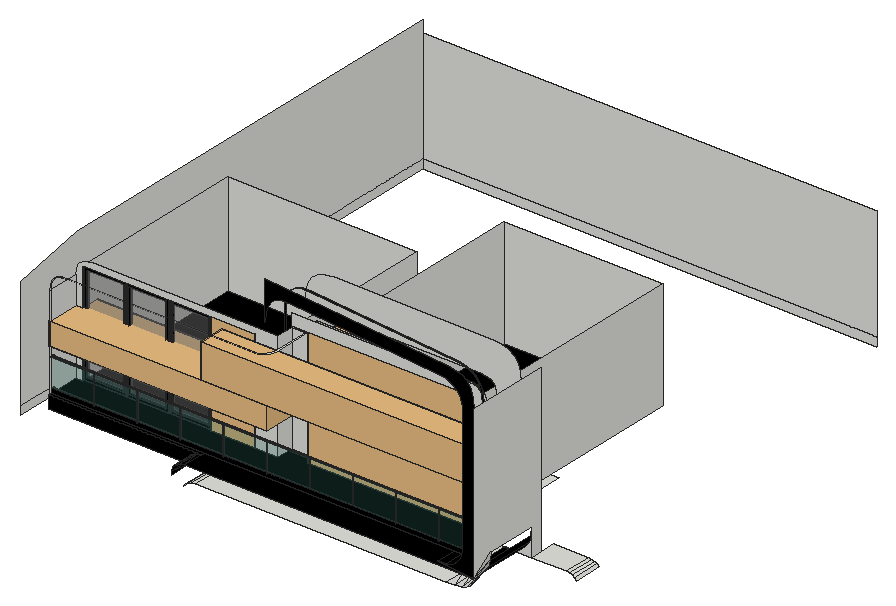
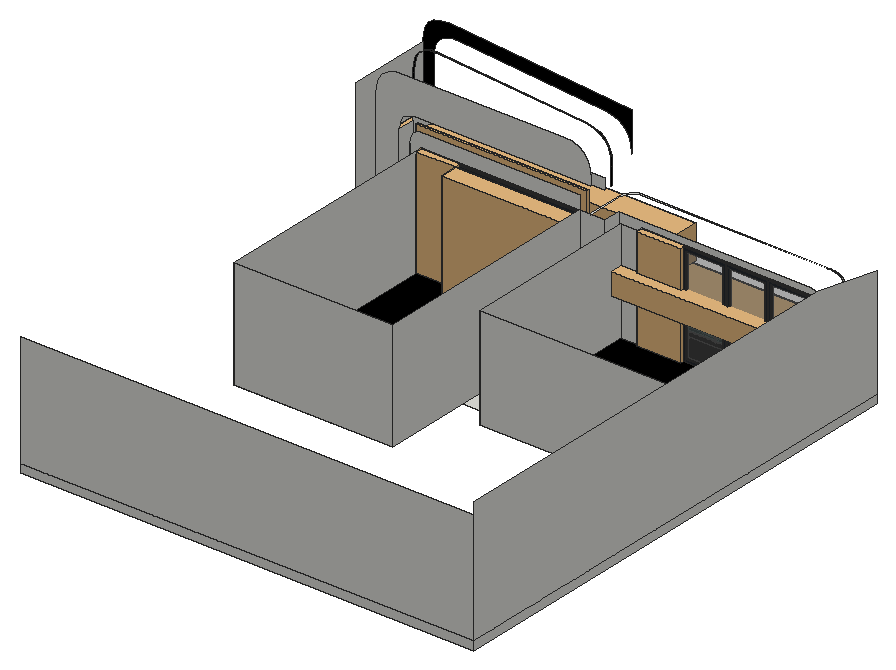
# SketchUp Ruby script. Lengths in inches.
U = 1.inch
M = Sketchup.active_model
def pt(a) = Geom::Point3d.new(a.map { |v| v * U })
def face(e, loops, mat)
  f = e.add_face(loops[0].map { |a| pt(a) })
  loops[1..].each { |l| e.add_face(l.map { |a| pt(a) }).erase! }
  f.material = f.back_material = mat if mat
  f
end
# faces: each face lists its corners as indices into pts; further lists are holes
def faces(e, pts, list, mat = nil) = list.each { |f| face(e, (f[0].is_a?(Array) ? f : [f]).map { |l| l.map { |i| pts[i] } }, mat) }
# xy, xz, yz: faces in a plane at the given z, y or x. An outline is a flat list of corners, or four numbers for a rectangle; further outlines are holes
def ring(l) = l.size == 4 ? [[l[0], l[1]], [l[2], l[1]], [l[2], l[3]], [l[0], l[3]]] : l.each_slice(2).to_a
def flat(e, list, mat, &to3) = list.each { |f| face(e, (f[0].is_a?(Array) ? f : [f]).map { |l| ring(l).map { |u, v| to3.(u, v) } }, mat) }
def xy(e, z, list, mat = nil) = flat(e, list, mat) { |x, y| [x, y, z] }
def xz(e, y, list, mat = nil) = flat(e, list, mat) { |x, z| [x, y, z] }
def yz(e, x, list, mat = nil) = flat(e, list, mat) { |y, z| [x, y, z] }
def lines(e, pts, list) = list.each { |a, b| e.add_line(pt(pts[a]), pt(pts[b])) }
# prism: a flat outline (further loops are holes) pulled along v
def prism(e, loops, v, mat = nil)
  f = face(e, loops, mat); d = Geom::Vector3d.new(v.map { |x| x * U })
  f.pushpull(f.normal.samedirection?(d) ? d.length : -d.length)
end
def box(e, o, s, mat = nil) = prism(e, [[o, [o[0] + s[0], o[1], o[2]], [o[0] + s[0], o[1] + s[1], o[2]], [o[0], o[1] + s[1], o[2]]]], [0, 0, s[2]], mat)
def at(x, y, z, deg = 0) = Geom::Transformation.translation(pt([x, y, z])) * Geom::Transformation.rotation(ORIGIN, Z_AXIS, deg.degrees)
def axes(o, x, y, z) = Geom::Transformation.new([*x, 0, *y, 0, *z, 0, *pt(o).to_a, 1])
def part(name) = M.definitions.add(name)
# library, detail: a bought-in or finely detailed component or shape, given as its bounding box
def library(name, o, s) = part(name).tap { |d| box(d.entities, o, s) }
def detail(e, o, s) = box(e.add_group.entities, o, s)
def put(e, d, t, mat = nil) = e.add_instance(d, t).tap { |i| i.material = mat if mat }
def group(e, t, mat = nil) = e.add_group.tap { |g| g.transformation = t; g.material = mat if mat }.entities
root = M.entities
M.materials.add("Glass Railing Color").color = [198, 198, 198]
M.materials.add("Railing Glass").color = [63, 150, 137]
M.materials["Railing Glass"].alpha = 0.13
M.materials.add("[0130_Gainsboro]").color = [39, 45, 50]
M.materials.add("[Color M00]").color = [255, 255, 255]
M.materials.add("[Color M09]").color = [0, 0, 0]
M.materials.add("[Color M09]1").color = [0, 0, 0]
M.materials.add("[Translucent Glass Gray]1").color = [128, 128, 128]
M.materials["[Translucent Glass Gray]1"].alpha = 0.5
M.materials.add("[Wood Veneer 02]").color = [190, 128, 91]
c1 = library("door by lz",[5.91,-4.92,0],[35.43,6.61,78.74])
c2 = part("Glazed door panel")
xy(c2.entities,0,[[0,-0.98,43.07,0],[0,0,43.07,1.4]],"[0130_Gainsboro]")
xy(c2.entities,0.3,[[0.3,-1.43,42.77,-0.98]],"[0130_Gainsboro]")
xy(c2.entities,2.95,[[2.95,-0.63,40.12,0],[2.95,0,40.12,0.64],[2.95,0.64,40.12,1.4]],"[0130_Gainsboro]")
xy(c2.entities,2.95,[[2.95,-1.43,40.12,-0.63]],"[Color M09]")
xy(c2.entities,3.54,[[3.54,0,39.53,0.64]],"[0130_Gainsboro]")
xy(c2.entities,3.54,[[3.54,-0.63,39.53,0]],"[Color M09]")
xy(c2.entities,111.8125,[[3.54,0,39.53,0.64]],"[0130_Gainsboro]")
xy(c2.entities,111.8125,[[3.54,-0.63,39.53,0]],"[Color M09]")
xy(c2.entities,112.4,[[2.95,-0.63,40.12,0],[2.95,0,40.12,0.64],[2.95,0.64,40.12,1.4]],"[0130_Gainsboro]")
xy(c2.entities,112.4,[[2.95,-1.43,40.12,-0.63]],"[Color M09]")
xy(c2.entities,115.05,[[0.3,-1.43,42.77,-0.98]],"[0130_Gainsboro]")
xy(c2.entities,115.35,[[0,-0.98,43.07,0],[0,0,43.07,1.4]],"[0130_Gainsboro]")
xz(c2.entities,-1.43,[[[0.3,0.3,42.77,115.05],[2.95,2.95,40.12,112.4]]],"[Color M09]")
xz(c2.entities,-0.98,[[[0,0,43.07,115.35],[0.3,0.3,42.77,115.05]]],"[Color M00]")
xz(c2.entities,-0.63,[[[2.95,2.95,40.12,112.4],[3.54,3.54,39.53,111.8125]]],"[Color M09]")
xz(c2.entities,0,[[[0,0,43.07,115.35],[2.95,2.95,40.12,112.4]],[[2.95,2.95,40.12,112.4],[3.54,3.54,39.53,111.8125]]],"[0130_Gainsboro]")
xz(c2.entities,0,[[3.54,3.54,39.53,111.8125]],"[Translucent Glass Gray]1")
xz(c2.entities,0.64,[[[2.95,2.95,40.12,112.4],[3.54,3.54,39.53,111.8125]]],"[0130_Gainsboro]")
xz(c2.entities,1.4,[[[0,0,43.07,115.35],[2.95,2.95,40.12,112.4]]],"[0130_Gainsboro]")
yz(c2.entities,0,[[-0.98,0,0,115.35],[0,0,1.4,115.35]],"[0130_Gainsboro]")
yz(c2.entities,0.3,[[-1.43,0.3,-0.98,115.05]],"[Color M00]")
yz(c2.entities,2.95,[[-0.63,2.95,0,112.4],[0,2.95,0.64,112.4],[0.64,2.95,1.4,112.4]],"[0130_Gainsboro]")
yz(c2.entities,2.95,[[-1.43,2.95,-0.63,112.4]],"[Color M09]")
yz(c2.entities,3.54,[[0,3.54,0.64,111.8125]],"[0130_Gainsboro]")
yz(c2.entities,3.54,[[-0.63,3.54,0,111.8125]],"[Color M09]")
yz(c2.entities,39.53,[[0,3.54,0.64,111.8125]],"[0130_Gainsboro]")
yz(c2.entities,39.53,[[-0.63,3.54,0,111.8125]],"[Color M09]")
yz(c2.entities,40.12,[[-0.63,2.95,0,112.4],[0,2.95,0.64,112.4],[0.64,2.95,1.4,112.4]],"[0130_Gainsboro]")
yz(c2.entities,40.12,[[-1.43,2.95,-0.63,112.4]],"[Color M09]")
yz(c2.entities,42.77,[[-1.43,0.3,-0.98,115.05]],"[Color M00]")
yz(c2.entities,43.07,[[-0.98,0,0,115.35],[0,0,1.4,115.35]],"[0130_Gainsboro]")
c3 = part("Sliding glass doors")
put(c3.entities,c2,axes([90.57,1.43,0],[1.05148,0,0],[0,1,0],[0,0,1]),"[Color M09]")
put(c3.entities,c2,axes([0,1.43,0],[1.05148,0,0],[0,1,0],[0,0,1]))
put(c3.entities,c2,axes([45.29,1.43,0],[1.05148,0,0],[0,1,0],[0,0,1]))
c4 = library("Curtains",[0,0,0],[121.73,8.19,117.22])
c5 = part("Glass Rail Spacer")
box(c5.entities,[-0.5,-0.25,0],[1,0.5,1],"Glass Railing Color")
c6 = part("Group242\#1")
xz(c6.entities,0,[[-0.01,0,0.18,0.02,0.37,0.09,0.52,0.21,0.64,0.37,0.72,0.54,0.75,0.74,0.73,0.93,0.66,1.12,0.54,1.27,0.38,1.39,0.21,1.47,0.01,1.5,-0.18,1.48,-0.37,1.41,-0.52,1.29,-0.64,1.13,-0.72,0.96,-0.75,0.76,-0.73,0.57,-0.66,0.38,-0.54,0.23,-0.38,0.11,-0.21,0.03]],"Glass Railing Color")
xz(c6.entities,457,[[-0.01,0,-0.21,0.03,-0.38,0.11,-0.54,0.23,-0.66,0.38,-0.73,0.57,-0.75,0.76,-0.72,0.96,-0.64,1.13,-0.52,1.29,-0.37,1.41,-0.18,1.48,0.01,1.5,0.21,1.47,0.38,1.39,0.54,1.27,0.66,1.12,0.73,0.93,0.75,0.74,0.72,0.54,0.64,0.37,0.52,0.21,0.37,0.09,0.18,0.02]],"Glass Railing Color")
p = [[-0.38,0,0.11],[-0.38,457,0.11],[-0.21,457,0.03],[-0.21,0,0.03],[-0.01,457,0],[-0.01,0,0],
  [0.18,457,0.02],[0.18,0,0.02],[0.37,457,0.09],[0.37,0,0.09],[-0.54,0,0.23],[-0.54,457,0.23],
  [0.52,457,0.21],[0.52,0,0.21],[-0.66,0,0.38],[-0.66,457,0.38],[0.64,457,0.37],[0.64,0,0.37],
  [-0.73,0,0.57],[-0.73,457,0.57],[0.72,457,0.54],[0.72,0,0.54],[0.75,457,0.74],[0.75,0,0.74],
  [-0.75,0,0.76],[-0.75,457,0.76],[0.73,457,0.93],[0.73,0,0.93],[-0.72,0,0.96],[-0.72,457,0.96],
  [0.66,457,1.12],[0.66,0,1.12],[-0.64,0,1.13],[-0.64,457,1.13],[-0.52,0,1.29],[-0.52,457,1.29],
  [0.54,457,1.27],[0.54,0,1.27],[-0.37,0,1.41],[-0.37,457,1.41],[0.38,457,1.39],[0.38,0,1.39],
  [-0.18,0,1.48],[-0.18,457,1.48],[0.21,457,1.47],[0.21,0,1.47],[0.01,0,1.5],[0.01,457,1.5]]
faces(c6.entities,p,[[0,1,2,3],[3,2,4,5],[5,4,6,7],[7,6,8,9],[10,11,1,0],[9,8,12,13],[14,15,11,10],[13,12,16,17],
  [18,19,15,14],[17,16,20,21],[21,20,22,23],[24,25,19,18],[23,22,26,27],[28,29,25,24],[27,26,30,31],[32,33,29,28],
  [34,35,33,32],[31,30,36,37],[38,39,35,34],[37,36,40,41],[42,43,39,38],[41,40,44,45],[46,47,43,42],[45,44,47,46]],"[Color M09]1")
c7 = part("Group245\#1")
prism(c7.entities,[[[0.25,0,5],[0.25,0,4],[-0.25,0,4],[-0.25,0,5],[-0.5,0,5],[-0.5,0,0],[0.5,0,0],[0.5,0,5]]],[0,457,0],"[Color M09]1")
c8 = part("Group246\#1")
box(c8.entities,[-0.1875,0,0],[0.375,44.6,30],"Railing Glass")
c9 = part("Group247\#1")
box(c9.entities,[-0.1875,0,0],[0.375,44.6,30],"Railing Glass")
c10 = part("Group248\#1")
box(c10.entities,[-0.1875,0,0],[0.375,44.6,30],"Railing Glass")
c11 = part("Group249\#1")
box(c11.entities,[-0.1875,0,0],[0.375,44.6,30],"Railing Glass")
c12 = part("Group250\#1")
box(c12.entities,[-0.1875,0,0],[0.375,44.6,30],"Railing Glass")
c13 = part("Group251\#1")
box(c13.entities,[-0.1875,0,0],[0.375,44.6,30],"Railing Glass")
c14 = part("Group252\#1")
box(c14.entities,[-0.1875,0,0],[0.375,44.6,30],"Railing Glass")
c15 = part("Group253\#1")
box(c15.entities,[-0.1875,0,0],[0.375,44.6,30],"Railing Glass")
c16 = part("Group254\#1")
box(c16.entities,[-0.1875,0,0],[0.375,44.6,30],"Railing Glass")
c17 = part("Group255\#1")
box(c17.entities,[-0.1875,0,0],[0.375,44.6,30],"Railing Glass")
c18 = part("Glass Railing")
put(c18.entities,c5,at(0,0,4))
put(c18.entities,c5,at(45.6,0,4))
put(c18.entities,c5,at(91.2,0,4))
put(c18.entities,c5,at(136.8,0,4))
put(c18.entities,c5,at(182.4,0,4))
put(c18.entities,c5,at(228,0,4))
put(c18.entities,c5,at(273.6,0,4))
put(c18.entities,c5,at(319.2,0,4))
put(c18.entities,c5,at(364.8,0,4))
put(c18.entities,c5,at(410.4,0,4))
put(c18.entities,c5,at(456,0,4))
put(c18.entities,c6,at(-0.5,0,34,-90),"Glass Railing Color")
put(c18.entities,c7,at(-0.5,0,0,-90),"Glass Railing Color")
put(c18.entities,c8,at(0.5,0,4,-90),"Railing Glass")
put(c18.entities,c9,at(46.1,0,4,-90),"Railing Glass")
put(c18.entities,c10,at(91.7,0,4,-90),"Railing Glass")
put(c18.entities,c11,at(137.3,0,4,-90),"Railing Glass")
put(c18.entities,c12,at(182.9,0,4,-90),"Railing Glass")
put(c18.entities,c13,at(228.5,0,4,-90),"Railing Glass")
put(c18.entities,c14,at(274.1,0,4,-90),"Railing Glass")
put(c18.entities,c15,at(319.7,0,4,-90),"Railing Glass")
put(c18.entities,c16,at(365.3,0,4,-90),"Railing Glass")
put(c18.entities,c17,at(410.9,0,4,-90),"Railing Glass")
c19 = library("Mesh Light",[-0.5,-0.5,-0.1],[1,1,0.2])
c20 = library("Group\#5",[-0.5,-0.5,0],[180.91,2,130.125])
c21 = library("Mesh Light\#1",[-0.5,-0.5,-0.1],[1,1,0.2])
xy(root,143.7,[[967.75,260.875,1015.75,406.0625],[1027.75,260.875,1183.9375,406.0625]])
xy(root,144,[[795.4375,260.875,931.4375,467.3125]])
xy(root,150,[[963.61,202.125,1228.2,233.0625],[1228,233.0625,1228.2,234.0625],[963.61,234.0625,963.61,260.875,1196.71,260.875,1196.71,278.875,1228.2,278.875,1228.2,234.0625],[1257.4375,278.875,1294.21,307.9375]])
xy(root,150,[[789.4375,224.875,937.4375,260.875]],"[Color M09]")
xy(root,163.875,[[951.61,202.125,1257.4375,202.125,1216.2,206.05,1216.2,231.99,952.57,231.99,952.57,224.875,951.61,224.875],[789.4375,224.875,951.61,224.875,951.61,232.99,1216.2,232.99,1216.2,260.875,1209.4375,260.875,1209.4375,278.875,1197.4375,278.875,1197.4375,527.4375,1029.53,527.4375,1029.53,278.875,1003.53,278.875,1003.53,260.875,978.47,260.875,978.47,266.1,996.66,266.1,996.66,453.4375,796.3125,453.4375,796.3125,260.875,789.4375,260.875]],"[Color M09]")
xz(root,224.875,[[789.4375,150,937.4375,150,937.83,154.24,939.01,157.71,940.98,160.41,943.74,162.33,947.28,163.49,951.61,163.875,789.4375,163.875]],"[Color M09]")
xz(root,260.875,[[789.4375,163.875,796.3125,163.875,796.3125,272.125,978.47,272.125,978.47,163.875,1003.53,163.875,1003.53,279,806.73,279,801.45,278.52,797.125,277.08,793.76,274.68,791.36,271.3125,789.92,266.99,789.4375,261.71],[1209.4375,163.875,1216.2,163.875,1221.4375,164.35,1221.4375,288.5625,1220.95,293.89,1219.5,298.25,1217.08,301.64,1213.6875,304.0625,1209.33,305.52,1204,306,1018.27,306,1018.27,294,1194.29,294,1198.92,293.58,1202.71,292.32,1205.65,290.21,1207.75,287.27,1209.02,283.48,1209.4375,278.86]])
xz(root,266.1,[[978.47,163.875,996.66,272.125]])
xz(root,278.875,[[1228.2,150,1257.4375,150,1257.4375,179.24,1256.625,170.31,1254.1875,163,1250.13,157.31,1244.44,153.25,1237.13,150.8125],[1003.53,163.875,1029.53,279],[1197.4375,163.875,1209.4375,163.875,1209.4375,278.86,1209.02,283.48,1207.75,287.27,1205.65,290.21,1202.71,292.32,1198.92,293.58,1194.29,294,1029.53,294,1029.53,279,1197.4375,279],[1216.2,163.875,1221.4375,163.875,1221.4375,164.35],[1221.4375,164.35,1225.13,164.6875,1232.44,167.125,1238.13,171.19,1242.1875,176.87,1244.625,184.18,1245.4375,193.12,1245.4375,312.76,1244.625,321.69,1242.1875,329,1238.13,334.69,1232.44,338.75,1225.13,341.1875,1216.2,342,1047.51,342,1038.58,341.1875,1031.27,338.75,1025.58,334.69,1021.52,329,1019.09,321.69,1018.27,312.76,1018.27,306,1204,306,1209.33,305.52,1213.6875,304.0625,1217.08,301.64,1219.5,298.25,1220.95,293.89,1221.4375,288.5625]])
xz(root,453.4375,[[796.3125,163.875,996.66,272.125]])
xz(root,527.4375,[[1029.53,163.875,1197.4375,279]])
xz(root,734.875,[[777.4375,150,1257.4375,159],[777.4375,159,1257.4375,279]])
yz(root,777.4375,[[202.125,150,734.875,159],[202.125,159,202.125,276.71,278.875,291,734.875,291,734.875,159]])
yz(root,789.4375,[[227.5,163.875,260.875,261.71]])
yz(root,796.3125,[[260.875,163.875,453.4375,272.125]])
yz(root,978.47,[[260.875,163.875,266.1,272.125]])
yz(root,996.66,[[266.1,163.875,453.4375,272.125]])
yz(root,1003.53,[[260.875,163.875,278.875,279]])
yz(root,1029.53,[[278.875,163.875,527.4375,279]])
yz(root,1197.4375,[[278.875,163.875,527.4375,279]])
yz(root,1209.4375,[[260.875,163.875,268.8125,278.86],[269.8125,163.875,278.875,278.86]])
yz(root,1221.4375,[[260.875,164.35,278.875,288.5625]])
yz(root,1257.4375,[[278.875,150,290.7,150,290.7,324.76,202.125,324.76,202.125,163.875,224.875,179.24,278.875,179.24]])
p = [[951.01,202.125,143.7],[951.01,233.0625,143.7],[952.98,233.0625,146.46],[952.98,202.125,146.46],[952.98,260.875,146.46],[952.98,234.0625,146.46],
  [951.01,234.0625,143.7],[951.01,260.875,143.7],[1304.88,278.875,144.67],[1304.88,307.9375,144.67],[1303.21,307.9375,147],[1303.21,278.875,147],
  [955.74,233.0625,148.43],[955.74,202.125,148.43],[955.74,260.875,148.43],[955.74,234.0625,148.43],[1300.88,307.9375,148.67],[1300.88,278.875,148.67],
  [959.28,233.0625,149.61],[959.28,202.125,149.61],[959.28,260.875,149.61],[959.28,234.0625,149.61],[1297.88,307.9375,149.67],[1297.88,278.875,149.67],
  [963.61,233.0625,150],[963.61,202.125,150],[963.61,260.875,150],[963.61,234.0625,150],[937.4375,224.875,150],[937.4375,202.125,149.7],
  [937.83,202.125,154.03],[1294.21,307.9375,150],[1294.21,278.875,150],[937.83,224.875,154.24],[1228.2,202.125,150],[1228.2,224.875,150],
  [1237.13,202.125,150.39],[1237.13,224.875,150.8125],[1228.2,233.0625,150],[1228.2,234.0625,150],[1228.2,278.875,150],[1237.13,278.875,150.8125],
  [1244.44,202.125,151.54],[1244.44,224.875,153.25],[1244.44,278.875,153.25],[1250.13,202.125,153.47],[1250.13,224.875,157.31],[1250.13,278.875,157.31],
  [1254.1875,202.125,156.17],[939.01,202.125,157.58],[939.01,224.875,157.71],[1254.1875,224.875,163],[1256.625,202.125,159.64],[1254.1875,278.875,163],
  [940.98,202.125,160.33],[940.98,224.875,160.41],[1256.625,224.875,170.31],[1257.4375,202.125,163.875],[943.74,202.125,162.3],[943.74,224.875,162.33],
  [947.28,202.125,163.48],[947.28,224.875,163.49],[1256.625,278.875,170.31],[951.61,202.125,163.875],[951.61,224.875,163.875],[1257.4375,202.125,324.76],
  [1256.625,202.2,333.69],[1254.1875,202.43,341],[1250.13,202.82,346.69],[1244.44,203.36,350.75],[1237.13,204.06,353.1875],[1228.2,204.91,354],
  [1018.27,224.875,354],[1018.27,224.875,312.76],[1019.09,224.8,321.69],[1021.52,224.57,329],[1025.58,224.18,334.69],[1031.27,223.64,338.75],
  [1038.58,222.94,341.1875],[1047.51,222.09,342],[1216.2,206.05,342],[1225.13,205.2,341.1875],[1232.44,204.5,338.75],[1238.13,203.96,334.69],
  [1242.1875,203.58,329],[1244.625,203.34,321.69],[1245.4375,203.27,312.76],[1245.4375,203.27,193.12],[1244.625,203.34,184.18],[1242.1875,203.58,176.87],
  [1238.13,203.96,171.19],[1232.44,204.5,167.125],[1225.13,205.2,164.6875],[1216.2,206.05,163.875],[1257.4375,224.875,179.24],[1225.13,231.14,164.6875],
  [1216.2,231.99,163.875],[1216.2,260.875,163.875],[1216.2,232.99,163.875],[1225.13,232.14,164.6875],[1225.13,278.875,164.6875],[1221.4375,278.875,164.35],
  [1221.4375,260.875,164.35],[1216.2,278.875,163.875],[1232.44,230.44,167.125],[1232.44,231.44,167.125],[1232.44,278.875,167.125],[789.4375,226.5,150],
  [789.4375,226.5,163.875],[789.4375,227.5,150],[789.4375,227.5,163.875]]
faces(root,p,[[0,1,2,3],[4,5,6,7],[8,9,10,11],[3,2,12,13],[14,15,5,4],[11,10,16,17],[13,12,18,19],[20,21,15,14],
  [17,16,22,23],[19,18,24,25],[26,27,21,20],[23,22,31,32],[34,35,36],[35,37,36],[36,37,42],[37,43,42],
  [42,43,45],[43,46,45],[45,46,48],[46,51,48],[48,51,52],[51,56,52],[52,56,57],[56,94,57],
  [101,103,97,102]])
faces(root,p,[[28,29,30],[33,28,30],[37,35,38,39,40,41],[43,37,41,44],[46,43,44,47],[33,30,49],[50,33,49],[51,46,47,53],
  [50,49,54],[55,50,54],[55,54,58],[59,55,58],[59,58,60],[61,59,60],[56,51,53,62],[61,60,63],
  [64,61,63],[65,66,67,68,69,70,71,72,73,74,75,76,77,78,79,80,81,82,83,84,85,86,87,88,89,90,91,92,93,57],[92,95,96,93],[97,98,99,100,101,102],[91,104,95,92],[100,99,105,106]],"[Color M09]")
lines(root,p,[[107,108],[109,110]])
put(root,c1,axes([924.08,266.36,163.875],[1.31569,0,0],[0,1,0],[0,0,1.37477]))
put(root,c3,axes([796.3125,262.25,163.875],[1,0,0],[0,1,0],[0,0,0.93841]))
put(root,c4,axes([1029.98,286.64,163.875],[1.02716,0,0],[0,2.19584,0],[0,0,0.98437]))
put(root,c1,axes([1147.93,284.36,163.875],[1.19735,0,0],[0,1,0],[0,0,1.46209]),"[Wood Veneer 02]")
put(root,c3,axes([1029.53,280.25,163.875],[0.92359,0,0],[0,1,0],[0,0,0.99801]))
put(root,c18,at(789.4375,228.54,163.875))
g1 = group(root,at(789.4375,226.5,163.875))
xy(g1,115.125,[[17.29,0,17.29,1,220.39,1,221.41,1.65,222.39,2.37,223.3125,3.15,224.18,4,224.98,4.91,225.71,5.875,226.375,6.89,226.96,7.94,227.48,9.04,227.91,10.17,228.26,11.33,228.53,12.51,228.53,52.375,229.53,52.375,229.53,12.51,229.29,11.19,228.9375,9.89,228.48,8.63,227.93,7.41,227.27,6.23,226.52,5.11,225.6875,4.0625,224.77,3.08,223.77,2.18,222.7,1.36,221.57,0.63,220.39,0]])
yz(g1,0,[[0,0,1,97.83]])
p = [[0,0,97.83],[0,1,97.83],[0.48,1,103.12],[0.48,0,103.12],[1.92,1,107.4375],[1.92,0,107.4375],
  [4.32,1,110.8],[4.32,0,110.8],[7.6875,1,113.2],[7.6875,0,113.2],[12.01,1,114.64],[12.01,0,114.64],
  [17.29,1,115.125],[17.29,0,115.125]]
faces(g1,p,[[0,1,2,3],[3,2,4,5],[5,4,6,7],[7,6,8,9],[9,8,10,11],[11,10,12,13]])
put(g1,c19,axes([114.77,26.1875,57.5625],[230.5313,0,0],[0,53.375,0],[0,0,116.125]))
put(root,c20,at(1029.53,268.8125,163.875))
g2 = group(root,at(951.61,224.875,163.875),"[Color M09]")
xy(g2,0,[[0,0,0.96,0,0.96,7.11,264.59,7.11,264.59,8.11,0,8.11]])
xy(g2,178.125,[[264.59,7.11,95.91,23.16,95.91,24.16,264.59,8.11]])
yz(g2,66.67,[[25.9375,130.125,26.9375,148.88]])
yz(g2,293.83,[[4.33,29.24,5.33,148.88]])
p = [[273.52,6.26,0.8125],[273.52,7.26,0.8125],[264.59,8.11,0],[264.59,7.11,0],[280.83,5.57,3.25],[280.83,6.57,3.25],
  [286.52,5.02,7.31],[286.52,6.02,7.31],[290.58,4.64,13],[290.58,5.64,13],[293.02,4.41,20.31],[293.02,5.41,20.31],
  [293.83,4.33,29.24],[293.83,5.33,29.24],[293.02,4.41,157.82],[293.02,5.41,157.82],[293.83,5.33,148.88],[293.83,4.33,148.88],
  [66.67,25.9375,148.88],[66.67,26.9375,148.88],[67.48,26.86,157.82],[67.48,25.86,157.82],[290.58,4.64,165.13],[290.58,5.64,165.13],
  [69.91,26.63,165.13],[69.91,25.63,165.13],[286.52,5.02,170.81],[286.52,6.02,170.81],[73.98,26.24,170.81],[73.98,25.24,170.81],
  [280.83,5.57,174.875],[280.83,6.57,174.875],[79.66,25.7,174.875],[79.66,24.7,174.875],[273.52,6.26,177.3125],[273.52,7.26,177.3125],
  [86.97,25.01,177.3125],[86.97,24.01,177.3125],[264.59,7.11,178.125],[264.59,8.11,178.125],[95.91,24.16,178.125],[95.91,23.16,178.125]]
faces(g2,p,[[0,1,2,3],[4,5,1,0],[6,7,5,4],[8,9,7,6],[10,11,9,8],[12,13,11,10],[14,15,16,17],[18,19,20,21],
  [22,23,15,14],[21,20,24,25],[26,27,23,22],[25,24,28,29],[30,31,27,26],[29,28,32,33],[34,35,31,30],[33,32,36,37],
  [38,39,35,34],[37,36,40,41]])
put(g2,c21,axes([146.91,13.47,89.0625],[294.82897,0,0],[0,27.9375,0],[0,0,179.125]))
